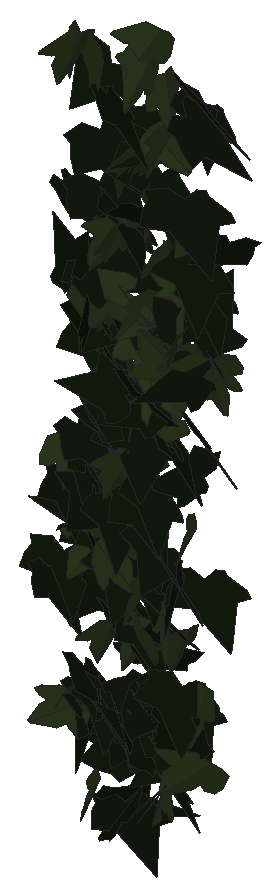
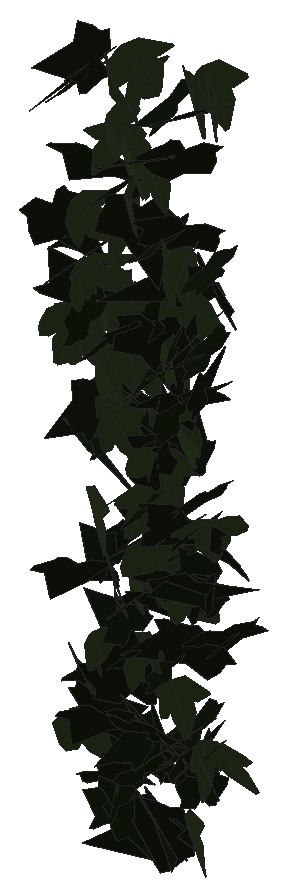
# SketchUp Ruby script. Lengths in inches.
U = 1.inch
M = Sketchup.active_model
def pt(a) = Geom::Point3d.new(a.map { |v| v * U })
def face(e, loops, mat)
  f = e.add_face(loops[0].map { |a| pt(a) })
  loops[1..].each { |l| e.add_face(l.map { |a| pt(a) }).erase! }
  f.material = f.back_material = mat if mat
  f
end
# faces: each face lists its corners as indices into pts; further lists are holes
def faces(e, pts, list, mat = nil) = list.each { |f| face(e, (f[0].is_a?(Array) ? f : [f]).map { |l| l.map { |i| pts[i] } }, mat) }
# xy, xz, yz: faces in a plane at the given z, y or x. An outline is a flat list of corners, or four numbers for a rectangle; further outlines are holes
def ring(l) = l.size == 4 ? [[l[0], l[1]], [l[2], l[1]], [l[2], l[3]], [l[0], l[3]]] : l.each_slice(2).to_a
def flat(e, list, mat, &to3) = list.each { |f| face(e, (f[0].is_a?(Array) ? f : [f]).map { |l| ring(l).map { |u, v| to3.(u, v) } }, mat) }
def xy(e, z, list, mat = nil) = flat(e, list, mat) { |x, y| [x, y, z] }
def xz(e, y, list, mat = nil) = flat(e, list, mat) { |x, z| [x, y, z] }
def yz(e, x, list, mat = nil) = flat(e, list, mat) { |y, z| [x, y, z] }
def lines(e, pts, list) = list.each { |a, b| e.add_line(pt(pts[a]), pt(pts[b])) }
# prism: a flat outline (further loops are holes) pulled along v
def prism(e, loops, v, mat = nil)
  f = face(e, loops, mat); d = Geom::Vector3d.new(v.map { |x| x * U })
  f.pushpull(f.normal.samedirection?(d) ? d.length : -d.length)
end
def box(e, o, s, mat = nil) = prism(e, [[o, [o[0] + s[0], o[1], o[2]], [o[0] + s[0], o[1] + s[1], o[2]], [o[0], o[1] + s[1], o[2]]]], [0, 0, s[2]], mat)
def at(x, y, z, deg = 0) = Geom::Transformation.translation(pt([x, y, z])) * Geom::Transformation.rotation(ORIGIN, Z_AXIS, deg.degrees)
def axes(o, x, y, z) = Geom::Transformation.new([*x, 0, *y, 0, *z, 0, *pt(o).to_a, 1])
def part(name) = M.definitions.add(name)
# library, detail: a bought-in or finely detailed component or shape, given as its bounding box
def library(name, o, s) = part(name).tap { |d| box(d.entities, o, s) }
def detail(e, o, s) = box(e.add_group.entities, o, s)
def put(e, d, t, mat = nil) = e.add_instance(d, t).tap { |i| i.material = mat if mat }
def group(e, t, mat = nil) = e.add_group.tap { |g| g.transformation = t; g.material = mat if mat }.entities
root = M.entities
M.materials.add("1026 AP 7946 SUNNY SIDE UP").color = [254, 231, 186]
M.materials.add("efeu1").color = [18, 25, 13]
M.materials.add("efeu2").color = [43, 57, 29]
c1 = part("ivyleaf_10")
p = [[0,0.5,-0.03],[-0.0625,2.02,-0.43],[-0.19,2.01,-0.46],[-0.54,1.05,-0.29],[-0.52,0.625,-0.18],[-0.83,0.76,-0.28],
  [-1.16,0.64,-0.33],[-1.15,0.33,-0.24],[-0.77,-0.39,0.02],[-0.3,-0.51,0.16],[0.04,-0.48,0.23],[-0.02,2.01,-0.4375],
  [-0.06,2.01,-0.43],[0.04,-0.49,0.23],[0.67,-0.49,0.14],[1.38,0.36,-0.2],[1.375,0.51,-0.24],[0.81,0.65,-0.19],
  [0.62,0.59,-0.15],[0.6,1.09,-0.28],[0.5,1.23,-0.31]]
faces(c1.entities,p,[[0,1,2,3,4,5,6,7,8,9,10],[11,12,0,13,14,15,16,17,18,19,20]],"efeu2")
c2 = part("ivyleaf_9")
p = [[1.54,2.16,1.25],[1.36,2.04,1.19],[-0.21,0.99,0.68],[-0.71,1.11,0.82],[-0.85,0.86,0.67],[-0.8,0.17,0.21],
  [-0.9,-0.01,0.1],[-0.67,-0.16,-0.02],[-0.08,-0.08,-0.05],[-0.03,-0.6,-0.4],[0.65,-0.88,-0.66],[0.83,-0.6,-0.49],
  [1.29,-0.42,-0.43],[1.8125,-0.07,-0.26],[1.21,0.44,0.15]]
faces(c2.entities,p,[[0,1,2,3,4,5,6,7,8,9,10,11,12,13,14]],"efeu1")
put(root,c1,axes([119.3,211.86,269.33],[0.32023,-0.0729,-0.16424],[-0.2552,0.01227,-0.21987],[0.10258,0.25809,-0.0343]),"1026 AP 7946 SUNNY SIDE UP")
put(root,c2,axes([119.74,211.62,275.16],[-0.01778,-0.00226,0.32868],[0.13792,0.30694,0.00724],[-0.48238,0.08784,-0.01005]),"1026 AP 7946 SUNNY SIDE UP")
put(root,c1,axes([120.06,211.69,271.93],[0.01496,0.28329,0.16355],[-0.01283,0.15738,-0.29084],[-0.50924,0.00436,0.01213]),"1026 AP 7946 SUNNY SIDE UP")
put(root,c1,axes([120.45,212.02,271.5],[0.08787,-0.22072,0.19687],[0.07754,-0.18593,-0.23564],[0.45378,0.07451,0.00214]),"1026 AP 7946 SUNNY SIDE UP")
put(root,c2,axes([119.92,211.93,278.57],[0.2375,-0.27182,-0.00124],[-0.01693,-0.00637,-0.32013],[0.42707,0.15091,-0.012]),"1026 AP 7946 SUNNY SIDE UP")
put(root,c2,axes([120.03,212.05,274.13],[-0.2033,-0.00003,0.26565],[-0.2836,-0.20616,-0.09439],[0.28979,-0.20177,0.09399]),"1026 AP 7946 SUNNY SIDE UP")
put(root,c1,axes([121.43,211.96,269.08],[-0.30291,-0.13175,0.20255],[-0.22885,-0.13519,-0.24011],[0.29471,-0.24039,0.02174]),"1026 AP 7946 SUNNY SIDE UP")
put(root,c2,axes([120.01,212.05,268.98],[0.00771,-0.01094,0.29458],[0.04683,-0.28448,-0.0134],[0.44761,0.02995,-0.00367]),"1026 AP 7946 SUNNY SIDE UP")
put(root,c2,axes([118.95,211.92,271.1875],[0.13018,-0.2549,-0.08366],[-0.04906,0.0737,-0.27558],[0.41709,0.08823,-0.0063]),"1026 AP 7946 SUNNY SIDE UP")
put(root,c2,axes([119.92,212.08,272.34],[-0.04464,-0.28556,0.08997],[-0.00399,-0.08912,-0.29608],[0.47028,-0.02786,0.00603]),"1026 AP 7946 SUNNY SIDE UP")
put(root,c2,axes([121.14,211.98,277.41],[-0.21133,-0.20319,-0.20862],[0.29077,0.10802,-0.23883],[0.34318,-0.21665,0.07389]),"1026 AP 7946 SUNNY SIDE UP")
put(root,c2,axes([120.89,212.09,271.66],[0.08996,-0.18917,0.23894],[0.11921,-0.22041,-0.2048],[0.45662,0.09481,0.00639]),"1026 AP 7946 SUNNY SIDE UP")
put(root,c2,axes([120.21,211.95,268.11],[-0.20075,-0.13383,-0.22907],[0.31705,0.10356,-0.1835],[0.25529,-0.23384,0.04775]),"1026 AP 7946 SUNNY SIDE UP")
put(root,c1,axes([119.73,211.85,275.67],[-0.20261,-0.06589,-0.33451],[0.51744,0.01155,-0.13703],[0.0554,-0.3488,0.05654]),"1026 AP 7946 SUNNY SIDE UP")
put(root,c1,axes([120.77,212.02,271.15],[0.24693,-0.17839,0.18101],[0.21594,-0.11348,-0.2444],[0.33055,0.20739,0.02444]),"1026 AP 7946 SUNNY SIDE UP")
put(root,c2,axes([121.43,211.93,274.93],[-0.42324,0.11593,0.00815],[-0.02741,-0.02222,-0.30074],[-0.18058,-0.26835,0.02655]),"1026 AP 7946 SUNNY SIDE UP")
put(root,c2,axes([119.48,212.05,269.38],[-0.25234,0.006,-0.28568],[0.40458,-0.11653,-0.15666],[-0.16302,-0.29848,0.0534]),"1026 AP 7946 SUNNY SIDE UP")
put(root,c2,axes([119.49,211.6875,275.93],[-0.00984,0.09636,0.31078],[-0.11566,0.29248,-0.09628],[-0.4835,-0.07193,0.0167]),"1026 AP 7946 SUNNY SIDE UP")
put(root,c2,axes([120.51,212.09,272.84],[-0.0137,-0.29149,0.07366],[0.01002,-0.07335,-0.30073],[0.47244,-0.00689,0.00851]),"1026 AP 7946 SUNNY SIDE UP")
put(root,c2,axes([119.51,212.18,272.33],[-0.19596,-0.18267,0.21521],[-0.01899,-0.22627,-0.21152],[0.43717,-0.09171,0.08728]),"1026 AP 7946 SUNNY SIDE UP")
put(root,c1,axes([119.3,212,279.18],[-0.09341,-0.31666,0.06672],[-0.00206,-0.06744,-0.33212],[0.5088,-0.05841,0.0109]),"1026 AP 7946 SUNNY SIDE UP")
put(root,c1,axes([119.99,212.08,276.57],[-0.14784,-0.2339,0.18596],[-0.04513,-0.18268,-0.25845],[0.46366,-0.09236,0.03414]),"1026 AP 7946 SUNNY SIDE UP")
put(root,c2,axes([119.68,212.125,269.5],[-0.04124,-0.26692,0.08658],[0.00126,-0.086,-0.27666],[0.44074,-0.02473,0.00889]),"1026 AP 7946 SUNNY SIDE UP")
put(root,c2,axes([120.57,212.17,271.98],[-0.13456,-0.23515,0.15031],[-0.01343,-0.15178,-0.25572],[0.43605,-0.07724,0.03851]),"1026 AP 7946 SUNNY SIDE UP")
put(root,c1,axes([120.1,212.05,273.21],[-0.10079,-0.27569,0.10512],[-0.01609,-0.10388,-0.2919],[0.46281,-0.06365,0.01275]),"1026 AP 7946 SUNNY SIDE UP")
put(root,c1,axes([119.61,211.98,268.18],[0.16414,-0.26736,-0.02037],[-0.0103,0.01704,-0.29558],[0.42125,0.10459,0.00071]),"1026 AP 7946 SUNNY SIDE UP")
put(root,c2,axes([120.99,212.09,270.06],[-0.17787,-0.26353,-0.06015],[0.04205,0.05043,-0.29511],[0.42184,-0.11614,0.00405]),"1026 AP 7946 SUNNY SIDE UP")
put(root,c2,axes([120.25,211.75,267.98],[-0.04053,0.2214,0.23387],[-0.03588,0.22461,-0.2283],[-0.4959,-0.03435,-0.0026]),"1026 AP 7946 SUNNY SIDE UP")
put(root,c2,axes([119.44,212.18,273.56],[0.31394,-0.19601,-0.13291],[0.19407,-0.05467,0.28447],[-0.31269,-0.23072,0.04311]),"1026 AP 7946 SUNNY SIDE UP")
put(root,c1,axes([119.95,212,276.59],[0.06358,-0.29976,-0.04405],[0.00974,0.04223,-0.31113],[0.47565,0.0392,0.01226]),"1026 AP 7946 SUNNY SIDE UP")
put(root,c2,axes([119.12,212.13,272.56],[-0.23367,-0.09927,-0.22594],[0.37443,-0.02696,-0.15421],[0.04981,-0.26308,0.09928]),"1026 AP 7946 SUNNY SIDE UP")
put(root,c1,axes([120.82,211.95,276.63],[-0.01955,-0.29197,-0.11599],[0.07132,0.10815,-0.29786],[0.48591,-0.02762,0.03905]),"1026 AP 7946 SUNNY SIDE UP")
put(root,c1,axes([121.28,212.11,270.01],[0.37303,-0.17768,0.09496],[0.09352,-0.07555,-0.30482],[0.30131,0.24343,-0.02296]),"1026 AP 7946 SUNNY SIDE UP")
put(root,c2,axes([119.375,212.125,269.75],[0.24507,-0.31189,0.03137],[0.00515,-0.03436,-0.35917],[0.49301,0.1554,-0.01184]),"1026 AP 7946 SUNNY SIDE UP")
put(root,c2,axes([120.33,212.13,268.95],[0.03594,-0.2875,0.02661],[0.00453,0.02777,0.29723],[-0.4541,-0.02248,0.00507]),"1026 AP 7946 SUNNY SIDE UP")
put(root,c1,axes([120.51,212.13,275.6],[0.14211,0.19098,-0.22029],[-0.22499,-0.16553,-0.21448],[-0.39211,0.16419,0.04323]),"1026 AP 7946 SUNNY SIDE UP")
put(root,c1,axes([121.01,212.03,275.38],[0.10521,-0.28439,-0.02867],[-0.01767,0.02428,-0.30078],[0.44872,0.06764,-0.00512]),"1026 AP 7946 SUNNY SIDE UP")
put(root,c2,axes([121.26,211.91,278.72],[0.27036,-0.19305,-0.22556],[-0.11264,0.21717,-0.25523],[0.44361,0.1728,0.07266]),"1026 AP 7946 SUNNY SIDE UP")
put(root,c2,axes([119.43,212.24,269.26],[-0.11513,-0.19427,0.19167],[-0.00555,-0.19322,-0.20918],[0.42414,-0.05527,0.04929]),"1026 AP 7946 SUNNY SIDE UP")
put(root,c2,axes([120.32,212.12,273.65],[-0.33921,-0.1457,-0.16169],[0.2189,0.07234,-0.26729],[0.25463,-0.25628,0.01438]),"1026 AP 7946 SUNNY SIDE UP")
put(root,c2,axes([120.82,212.16,271.73],[-0.21209,0.03918,-0.26203],[0.36414,-0.10733,-0.14406],[-0.17727,-0.26736,0.01758]),"1026 AP 7946 SUNNY SIDE UP")
put(root,c2,axes([120.61,212.06,274.16],[-0.40854,0.12198,0.03967],[-0.07313,-0.01054,-0.29424],[-0.18702,-0.26234,0.02839]),"1026 AP 7946 SUNNY SIDE UP")
put(root,c1,axes([120.63,212.21,268.33],[-0.00187,0.09934,-0.2552],[0.00247,-0.24828,-0.10379],[-0.42048,-0.0019,0.00053]),"1026 AP 7946 SUNNY SIDE UP")
put(root,c2,axes([119.76,211.98,277.97],[0.01798,-0.22775,-0.2615],[0.00938,0.25278,-0.23309],[0.53464,0.00322,0.01288]),"1026 AP 7946 SUNNY SIDE UP")
put(root,c2,axes([119.6,212.21,269.1],[-0.07513,0.05011,0.28488],[-0.25159,-0.23512,0.01405],[0.36276,-0.15269,0.06875]),"1026 AP 7946 SUNNY SIDE UP")
put(root,c2,axes([120.24,212,268.86],[-0.40771,-0.08399,-0.11909],[-0.1868,-0.00461,0.27909],[-0.12375,0.28366,-0.02892]),"1026 AP 7946 SUNNY SIDE UP")
put(root,c2,axes([121.17,211.96,269.3],[0.04667,-0.01055,0.29805],[-0.29625,0.22019,0.02946],[-0.34575,-0.19009,0.01498]),"1026 AP 7946 SUNNY SIDE UP")
put(root,c2,axes([118.96,212.17,271.34],[-0.11008,-0.28729,-0.05747],[0.02929,0.05119,-0.30426],[0.45875,-0.0722,0.00563]),"1026 AP 7946 SUNNY SIDE UP")
put(root,c2,axes([121.14,212.2,276.41],[-0.11074,-0.3067,-0.01058],[0.01826,0.00608,-0.32399],[0.4821,-0.07068,0.00984]),"1026 AP 7946 SUNNY SIDE UP")
put(root,c2,axes([120.38,212.18,275.2],[0.28861,-0.24617,0.05945],[-0.02978,0.05944,0.31601],[-0.39696,-0.18344,0.01951]),"1026 AP 7946 SUNNY SIDE UP")
put(root,c1,axes([119.58,212.03,279.04],[0.30645,-0.23264,-0.09925],[-0.05049,0.09621,-0.30994],[0.3919,0.19431,0.03768]),"1026 AP 7946 SUNNY SIDE UP")
put(root,c1,axes([119.5,212.23,271.6875],[-0.20158,-0.16667,0.20179],[-0.02053,-0.21532,-0.19786],[0.40503,-0.09386,0.0904]),"1026 AP 7946 SUNNY SIDE UP")
put(root,c2,axes([119.65,211.89,276.08],[0.20181,-0.0573,-0.31269],[0.07506,0.32811,-0.04114],[0.47935,-0.02725,0.13809]),"1026 AP 7946 SUNNY SIDE UP")
put(root,c1,axes([119.92,212.22,273.49],[0.22252,-0.12845,0.21852],[0.24031,-0.14821,-0.1977],[0.3083,0.20823,-0.00362]),"1026 AP 7946 SUNNY SIDE UP")
put(root,c2,axes([120.06,212.23,271.55],[-0.25506,-0.23623,-0.00902],[0.01927,0.00058,-0.29504],[0.37113,-0.16238,0.00911]),"1026 AP 7946 SUNNY SIDE UP")
put(root,c1,axes([121,212.26,275.95],[-0.22528,-0.13392,0.23836],[-0.08108,-0.24453,-0.17955],[0.41352,-0.12091,0.09465]),"1026 AP 7946 SUNNY SIDE UP")
put(root,c2,axes([120.81,212.2,268.69],[-0.21251,0.08139,-0.22101],[0.20596,-0.17768,-0.15516],[-0.29705,-0.18143,0.05052]),"1026 AP 7946 SUNNY SIDE UP")
put(root,c2,axes([119.25,212.28,271.65],[-0.04475,-0.03314,0.30434],[0.06786,-0.29427,-0.03142],[0.46277,0.03995,0.03404]),"1026 AP 7946 SUNNY SIDE UP")
put(root,c2,axes([119.93,212.32,269.07],[-0.11944,-0.2198,0.17379],[-0.00899,-0.1749,-0.23671],[0.43678,-0.0637,0.04265]),"1026 AP 7946 SUNNY SIDE UP")
put(root,c1,axes([120.75,212.22,274.74],[-0.30868,-0.18047,-0.19741],[-0.24101,-0.11439,0.27355],[-0.33504,0.24855,-0.0149]),"1026 AP 7946 SUNNY SIDE UP")
put(root,c2,axes([119.9,212.29,276.71],[0.02813,-0.27229,0.13556],[0.07574,-0.12912,-0.27947],[0.47053,0.03706,0.03688]),"1026 AP 7946 SUNNY SIDE UP")
put(root,c2,axes([120.67,212.21,273.67],[0.19628,-0.25936,0.05823],[0.01925,-0.05839,-0.29651],[0.41744,0.12464,-0.01371]),"1026 AP 7946 SUNNY SIDE UP")
put(root,c1,axes([120.125,212.17,277.69],[0.01382,-0.30378,0.0517],[0.01485,-0.05165,-0.31328],[0.48436,0.01025,0.00813]),"1026 AP 7946 SUNNY SIDE UP")
put(root,c1,axes([120.2,212.32,278.98],[-0.08808,-0.18734,0.26386],[0.14108,-0.25985,-0.17638],[0.48002,0.04199,0.10026]),"1026 AP 7946 SUNNY SIDE UP")
put(root,c1,axes([119.21,212.09,279.11],[0.20019,-0.27793,-0.0589],[0.0239,0.06755,-0.31166],[0.44504,0.1214,0.04323]),"1026 AP 7946 SUNNY SIDE UP")
put(root,c2,axes([119.96,212.25,273.96],[0.10284,-0.09449,0.29718],[0.25365,-0.2398,-0.11978],[0.40527,0.17406,-0.00044]),"1026 AP 7946 SUNNY SIDE UP")
put(root,c2,axes([121.35,212.05,273.36],[-0.32061,0.22609,0.05045],[-0.07439,0.0214,-0.3128],[-0.35563,-0.2083,0.01995]),"1026 AP 7946 SUNNY SIDE UP")
put(root,c1,axes([120.05,212.14,272.05],[-0.42397,-0.16946,0.06238],[-0.05671,-0.05773,-0.32704],[0.27774,-0.27047,0.02844]),"1026 AP 7946 SUNNY SIDE UP")
put(root,c1,axes([121.14,212.07,272.44],[0.12126,-0.27448,-0.11683],[-0.05993,0.10543,-0.293],[0.46218,0.08569,-0.00734]),"1026 AP 7946 SUNNY SIDE UP")
put(root,c2,axes([120.43,212.26,270.93],[0.09152,-0.16789,0.21703],[0.21615,-0.16794,-0.17719],[0.36564,0.1413,0.05042]),"1026 AP 7946 SUNNY SIDE UP")
put(root,c2,axes([121.01,212.17,278.96],[0.38316,-0.18173,0.08195],[0.0792,-0.06687,-0.31268],[0.30239,0.24779,-0.02194]),"1026 AP 7946 SUNNY SIDE UP")
put(root,c2,axes([119.22,212.26,268.93],[0.33582,-0.18328,-0.0339],[0.07583,0.0077,0.28745],[-0.28251,-0.2158,0.03687]),"1026 AP 7946 SUNNY SIDE UP")
put(root,c1,axes([121.09,212.32,275.77],[-0.08736,-0.20133,0.22533],[0.11122,-0.22617,-0.19627],[0.45539,0.01661,0.09116]),"1026 AP 7946 SUNNY SIDE UP")
put(root,c1,axes([120.35,212.29,277.17],[0.1307,-0.22018,0.19972],[0.18298,-0.16162,-0.23989],[0.42486,0.13734,0.04188]),"1026 AP 7946 SUNNY SIDE UP")
put(root,c1,axes([120.62,212.26,278.17],[0.0567,-0.27824,0.13199],[0.04188,-0.12727,-0.28963],[0.48088,0.04389,0.00966]),"1026 AP 7946 SUNNY SIDE UP")
put(root,c2,axes([120.07,212.02,269.27],[-0.29658,0.23778,0.10581],[0.12048,-0.0684,0.3118],[0.38817,0.20291,-0.01593]),"1026 AP 7946 SUNNY SIDE UP")
put(root,c1,axes([121.44,212.17,275.0625],[-0.30528,-0.2195,0.01477],[0.00644,-0.02439,-0.30138],[0.34595,-0.19324,0.01865]),"1026 AP 7946 SUNNY SIDE UP")
put(root,c2,axes([120.21,212.22,272.59],[-0.00586,-0.27069,-0.11338],[0.008,0.10846,-0.27823],[0.4585,-0.00535,0.00341]),"1026 AP 7946 SUNNY SIDE UP")
put(root,c1,axes([119.42,212.4,276.44],[-0.04876,-0.06645,0.32875],[0.2778,-0.27325,-0.04249],[0.43143,0.16844,0.06451]),"1026 AP 7946 SUNNY SIDE UP")
put(root,c2,axes([121.17,212.375,278.65],[-0.03041,-0.29155,0.11067],[0.01182,-0.1097,-0.30132],[0.48933,-0.01547,0.01416]),"1026 AP 7946 SUNNY SIDE UP")
put(root,c1,axes([120.2,212.3125,270.5625],[-0.08949,-0.22279,0.16215],[0.02167,-0.16419,-0.23338],[0.42952,-0.03814,0.04556]),"1026 AP 7946 SUNNY SIDE UP")
put(root,c1,axes([119.43,212.34,274.15],[0.13517,-0.21953,0.19067],[0.09762,-0.17575,-0.24386],[0.44212,0.10593,-0.00445]),"1026 AP 7946 SUNNY SIDE UP")
put(root,c2,axes([121.26,212.03,275.42],[-0.33317,-0.0198,0.2682],[0.39365,0.08027,0.21657],[-0.11716,0.32601,-0.035]),"1026 AP 7946 SUNNY SIDE UP")
put(root,c2,axes([119.52,212.42,278.73],[-0.2621,-0.21835,0.14486],[-0.03515,-0.15581,-0.27504],[0.40792,-0.15372,0.06938]),"1026 AP 7946 SUNNY SIDE UP")
put(root,c1,axes([120.44,212.2,277.89],[0.09227,-0.30278,-0.02514],[-0.01669,0.02105,-0.31754],[0.47714,0.05929,-0.00624]),"1026 AP 7946 SUNNY SIDE UP")
put(root,c2,axes([120.29,212.32,269.59],[-0.42596,-0.07751,-0.04374],[0.07716,-0.01978,-0.28849],[0.11517,-0.27342,0.03153]),"1026 AP 7946 SUNNY SIDE UP")
put(root,c2,axes([119.72,212.3,270.625],[0.21351,-0.23517,0.06947],[0.04356,-0.06339,-0.28002],[0.3828,0.13838,-0.00688]),"1026 AP 7946 SUNNY SIDE UP")
put(root,c1,axes([120.3,212.11,270.65],[-0.32026,0.11664,0.19018],[-0.2851,0.04874,-0.23839],[-0.18977,-0.27008,0.03718]),"1026 AP 7946 SUNNY SIDE UP")
put(root,c2,axes([120.03,212.16,273.67],[-0.38242,-0.16324,0.07761],[0.08421,0.05683,0.30159],[-0.2705,0.24847,-0.01583]),"1026 AP 7946 SUNNY SIDE UP")
put(root,c2,axes([119.62,212.43,275.05],[-0.21275,-0.20911,0.16728],[-0.05722,-0.16725,-0.25225],[0.4135,-0.13073,0.05116]),"1026 AP 7946 SUNNY SIDE UP")
put(root,c2,axes([120.11,212.36,269.03],[0.08407,-0.16336,0.22721],[0.17422,-0.19375,-0.17591],[0.39612,0.11988,0.02915]),"1026 AP 7946 SUNNY SIDE UP")
put(root,c2,axes([119.875,212.03,267.99],[0.29489,0.09198,0.2284],[0.33162,0.06981,-0.21372],[-0.17861,0.28146,-0.01971]),"1026 AP 7946 SUNNY SIDE UP")
put(root,c2,axes([120.46,212.35,277.41],[0.00905,-0.30203,0.03192],[-0.00394,-0.03275,-0.31138],[0.47767,0.00545,-0.00318]),"1026 AP 7946 SUNNY SIDE UP")
put(root,c2,axes([121.18,212.36,276.04],[0.03367,-0.30882,0.03301],[0.00045,-0.03386,-0.3191],[0.48849,0.02131,-0.00198]),"1026 AP 7946 SUNNY SIDE UP")
put(root,c2,axes([120.3125,212.13,276.97],[0.13636,0.27176,-0.13104],[-0.05541,-0.12388,-0.29458],[-0.46959,0.09354,-0.00329]),"1026 AP 7946 SUNNY SIDE UP")
put(root,c1,axes([120.47,212.37,278.77],[0.27638,-0.08981,0.26371],[0.31852,-0.16033,-0.20178],[0.28486,0.26641,-0.03024]),"1026 AP 7946 SUNNY SIDE UP")
put(root,c1,axes([119.7,212.29,275.17],[0.03958,-0.28978,0.062],[0.01226,-0.06138,-0.3],[0.46574,0.02624,0.00263]),"1026 AP 7946 SUNNY SIDE UP")
put(root,c1,axes([121.33,212.21,274.92],[-0.42219,0.08682,-0.08],[0.09673,-0.06141,-0.28841],[-0.15614,-0.27281,0.03763]),"1026 AP 7946 SUNNY SIDE UP")
put(root,c2,axes([119.58,212.29,271.97],[-0.18309,-0.23853,-0.14621],[0.15244,0.10771,-0.2704],[0.40779,-0.14736,0.03544]),"1026 AP 7946 SUNNY SIDE UP")
put(root,c1,axes([119.24,212.16,269.48],[-0.05999,-0.2667,-0.10497],[0.02319,0.09929,-0.27697],[0.44748,-0.0409,0.00028]),"1026 AP 7946 SUNNY SIDE UP")
put(root,c2,axes([119.2,212.21,273.28],[0.13137,-0.23882,-0.14441],[-0.03682,0.13839,-0.25896],[0.43278,0.08426,0.02181]),"1026 AP 7946 SUNNY SIDE UP")
put(root,c2,axes([119.57,212.21,277.04],[-0.05268,-0.20485,-0.24033],[0.16032,0.21315,-0.2077],[0.45964,-0.09783,0.0449]),"1026 AP 7946 SUNNY SIDE UP")
put(root,c2,axes([120.18,212.41,271.51],[0.00318,-0.27949,0.08633],[0.00426,-0.08537,-0.28843],[0.4595,0.00273,0.00208]),"1026 AP 7946 SUNNY SIDE UP")
put(root,c1,axes([121.07,212.41,276.83],[-0.04881,-0.23961,0.20995],[0.03165,-0.20724,-0.24742],[0.495,-0.01038,0.03652]),"1026 AP 7946 SUNNY SIDE UP")
put(root,c1,axes([120.37,212.26,274.91],[0.43773,0.16,-0.00793],[0.00887,-0.02704,-0.32983],[-0.2518,0.2772,-0.02541]),"1026 AP 7946 SUNNY SIDE UP")
put(root,c2,axes([120.18,212.3125,270.7],[0.02,-0.27276,-0.06582],[-0.01211,0.06205,-0.2809],[0.43978,0.01411,-0.00474]),"1026 AP 7946 SUNNY SIDE UP")
put(root,c2,axes([119.87,212.375,273.48],[0.10739,-0.07352,0.29343],[0.22484,-0.24773,-0.10249],[0.40495,0.15704,-0.02091]),"1026 AP 7946 SUNNY SIDE UP")
put(root,c1,axes([119.59,212.42,276.46],[0.05726,-0.23939,0.20616],[0.12436,-0.18921,-0.24744],[0.47602,0.07823,0.03984]),"1026 AP 7946 SUNNY SIDE UP")
put(root,c1,axes([120.26,212.4,279.37],[-0.19671,-0.22135,0.18714],[-0.01023,-0.19728,-0.25169],[0.4514,-0.10093,0.07585]),"1026 AP 7946 SUNNY SIDE UP")
put(root,c1,axes([119,212.26,272.92],[0.28464,0.25615,-0.02967],[-0.00567,-0.03445,-0.32286],[-0.40554,0.18027,-0.01631]),"1026 AP 7946 SUNNY SIDE UP")
put(root,c2,axes([120.98,212.26,273.97],[0.38708,-0.1609,-0.02547],[-0.06108,-0.01622,-0.30095],[0.24836,0.24679,-0.03432]),"1026 AP 7946 SUNNY SIDE UP")
put(root,c2,axes([119.3125,212.19,271.07],[0.03827,-0.07129,-0.29919],[0.276,0.23883,-0.04391],[0.37992,-0.16632,0.06203]),"1026 AP 7946 SUNNY SIDE UP")
put(root,c2,axes([120.01,212.21,275.4],[0.15116,0.2301,-0.1641],[-0.13865,-0.13639,-0.25649],[-0.41887,0.12819,0.02568]),"1026 AP 7946 SUNNY SIDE UP")
put(root,c2,axes([120.5,212.28,268.3],[-0.18194,0.20935,-0.12014],[0.07291,-0.10884,-0.24681],[-0.37063,-0.12418,0.01043]),"1026 AP 7946 SUNNY SIDE UP")
put(root,c2,axes([119.01,212.4,275.46],[0.1818,-0.26186,0.08499],[0.04481,-0.0792,-0.2953],[0.43008,0.11895,-0.00516]),"1026 AP 7946 SUNNY SIDE UP")
put(root,c1,axes([119.9,212.32,273.59],[-0.39444,-0.1195,0.07264],[-0.06415,-0.07714,-0.28194],[0.2091,-0.24908,0.05053]),"1026 AP 7946 SUNNY SIDE UP")
put(root,c2,axes([119.46,212.41,274.7],[-0.1532,-0.28692,-0.07808],[0.06693,0.06371,-0.31115],[0.46114,-0.10457,0.01922]),"1026 AP 7946 SUNNY SIDE UP")
put(root,c2,axes([121.1875,212.34,271.61],[-0.12304,-0.23501,-0.16137],[0.10649,0.14076,-0.25377],[0.42994,-0.10212,0.01668]),"1026 AP 7946 SUNNY SIDE UP")
put(root,c2,axes([120.68,212.48,268.86],[-0.29901,-0.15985,0.10163],[-0.09852,-0.07972,-0.25562],[0.27924,-0.19929,0.01863]),"1026 AP 7946 SUNNY SIDE UP")
put(root,c1,axes([120.66,212.09,273.92],[0.15695,0.17405,-0.24589],[0.10976,0.23196,0.20485],[0.45263,-0.1166,0.03559]),"1026 AP 7946 SUNNY SIDE UP")
put(root,c2,axes([120.89,212.48,275.33],[0.17295,-0.23831,0.17038],[0.07542,-0.16096,-0.27053],[0.45107,0.11828,-0.02009]),"1026 AP 7946 SUNNY SIDE UP")
put(root,c2,axes([119.97,212.45,272.97],[0.14638,-0.26285,0.06901],[0.02418,-0.06717,-0.28755],[0.42641,0.09404,-0.00739]),"1026 AP 7946 SUNNY SIDE UP")
put(root,c2,axes([120.12,212.32,269.47],[0.35248,-0.16199,-0.02558],[-0.0418,0.00399,-0.28462],[0.25406,0.2254,-0.01134]),"1026 AP 7946 SUNNY SIDE UP")
put(root,c2,axes([121.51,212.39,276.74],[-0.04183,0.18389,-0.24059],[-0.01195,-0.23586,-0.19096],[-0.46854,-0.0104,0.02635]),"1026 AP 7946 SUNNY SIDE UP")
put(root,c2,axes([120.4375,212.48,268.44],[0.14553,-0.23314,0.14735],[0.09054,-0.13243,-0.25916],[0.42156,0.10893,0.00479]),"1026 AP 7946 SUNNY SIDE UP")
put(root,c2,axes([120.79,212.36,269.6],[-0.12067,-0.21452,-0.16757],[0.12599,0.14196,-0.23273],[0.40292,-0.10863,0.02258]),"1026 AP 7946 SUNNY SIDE UP")
put(root,c2,axes([120.25,212.27,275.37],[0.14955,-0.20551,-0.19843],[0.00979,0.20362,-0.22079],[0.44152,0.0651,0.07211]),"1026 AP 7946 SUNNY SIDE UP")
put(root,c2,axes([119.15,212.38,275.72],[0.17201,-0.26835,-0.0789],[-0.063,0.06466,-0.29789],[0.4336,0.11585,-0.01198]),"1026 AP 7946 SUNNY SIDE UP")
put(root,c2,axes([120.28,212.39,270.14],[0.38368,0.07404,0.14152],[-0.21987,-0.00774,0.26091],[0.10764,-0.27971,0.02849]),"1026 AP 7946 SUNNY SIDE UP")
put(root,c1,axes([119.96,212.25,274.66],[-0.26191,0.23627,0.08528],[-0.10779,0.05093,-0.29633],[-0.37789,-0.17828,0.02542]),"1026 AP 7946 SUNNY SIDE UP")
put(root,c2,axes([119.18,212.12,271.96],[0.20757,0.11053,0.23269],[0.22567,0.1755,-0.17435],[-0.32359,0.19329,0.02767]),"1026 AP 7946 SUNNY SIDE UP")
put(root,c2,axes([119.11,212.54,274.76],[-0.02096,0.0175,0.30444],[-0.19366,-0.26922,0.00913],[0.42313,-0.12235,0.01926]),"1026 AP 7946 SUNNY SIDE UP")
put(root,c2,axes([119.67,212.32,275.28],[0.31415,-0.19944,-0.13147],[-0.16345,0.0745,-0.28974],[0.33345,0.22442,-0.01816]),"1026 AP 7946 SUNNY SIDE UP")
put(root,c2,axes([118.89,212.34,276.73],[0.29343,-0.2246,-0.07793],[-0.03173,0.07927,-0.29831],[0.37066,0.18459,0.03616]),"1026 AP 7946 SUNNY SIDE UP")
put(root,c1,axes([120.63,212.47,274.6875],[0.05144,-0.25985,0.13088],[0.06612,-0.12371,-0.26943],[0.45101,0.04777,0.02457]),"1026 AP 7946 SUNNY SIDE UP")
put(root,c1,axes([120.4375,212.46,274],[-0.1409,-0.25326,0.12274],[-0.02278,-0.12224,-0.27629],[0.44047,-0.08734,0.02498]),"1026 AP 7946 SUNNY SIDE UP")
put(root,c2,axes([119.17,212.43,272.875],[0.09874,-0.27414,-0.045],[-0.02007,0.04029,-0.28948],[0.43566,0.06399,-0.00314]),"1026 AP 7946 SUNNY SIDE UP")
put(root,c1,axes([120,212.31,272.98],[-0.28856,-0.19788,-0.11388],[0.16471,0.05048,-0.27476],[0.31509,-0.20761,0.03934]),"1026 AP 7946 SUNNY SIDE UP")
put(root,c1,axes([119.54,212.39,270.36],[-0.09503,-0.28023,0.02481],[0.00016,-0.02628,-0.29543],[0.44249,-0.06018,0.00544]),"1026 AP 7946 SUNNY SIDE UP")
put(root,c2,axes([119.46,212.48,274.44],[0.26368,-0.24257,0.10155],[0.05193,-0.09816,-0.30308],[0.40924,0.16874,-0.02697]),"1026 AP 7946 SUNNY SIDE UP")
put(root,c1,axes([120.52,212.21,278.05],[0.15895,0.23385,0.1821],[0.04711,0.17637,-0.25894],[-0.45726,0.09946,0.03662]),"1026 AP 7946 SUNNY SIDE UP")
put(root,c1,axes([120.78,212.41,270.64],[-0.04454,-0.27641,0.03496],[0.00011,-0.03569,-0.28643],[0.4382,-0.02809,0.00362]),"1026 AP 7946 SUNNY SIDE UP")
put(root,c2,axes([120.28,212.61,277.87],[-0.33517,-0.172,0.14957],[-0.05801,-0.17179,-0.26469],[0.35015,-0.19311,0.09932]),"1026 AP 7946 SUNNY SIDE UP")
put(root,c2,axes([119.38,212.38,272.91],[-0.14849,-0.14086,-0.26234],[0.30237,0.16964,-0.16967],[0.34199,-0.21115,0.0361]),"1026 AP 7946 SUNNY SIDE UP")
put(root,c2,axes([119.55,212.46,271.85],[-0.18726,0.03869,0.26088],[-0.39833,-0.05775,-0.11408],[0.05758,-0.27361,0.05926]),"1026 AP 7946 SUNNY SIDE UP")
